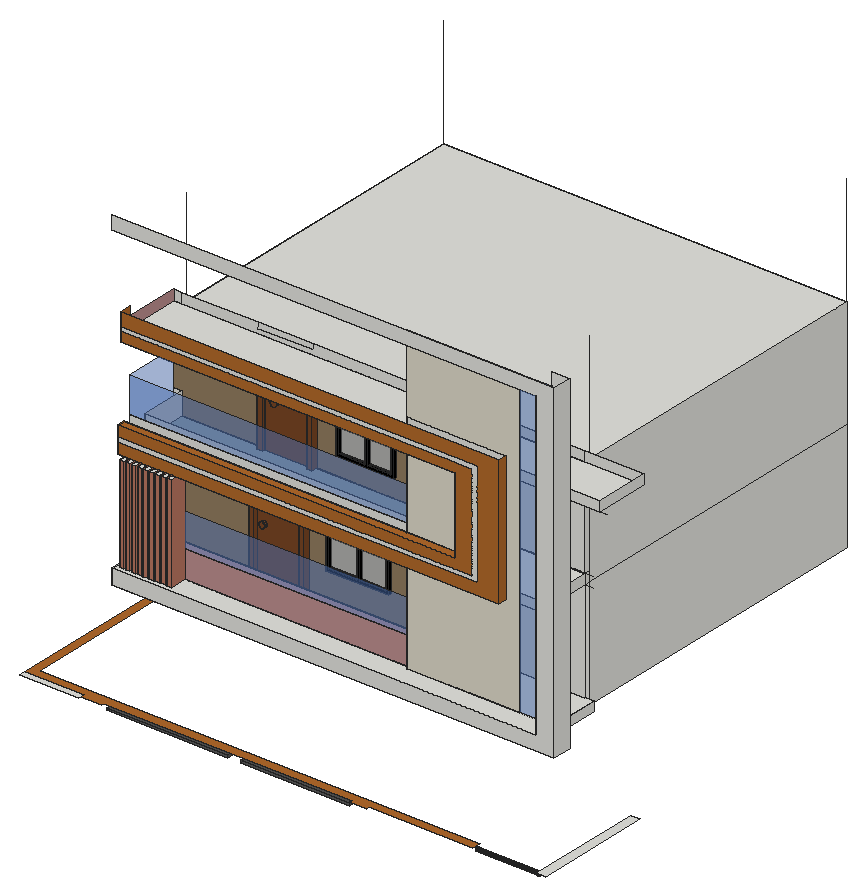
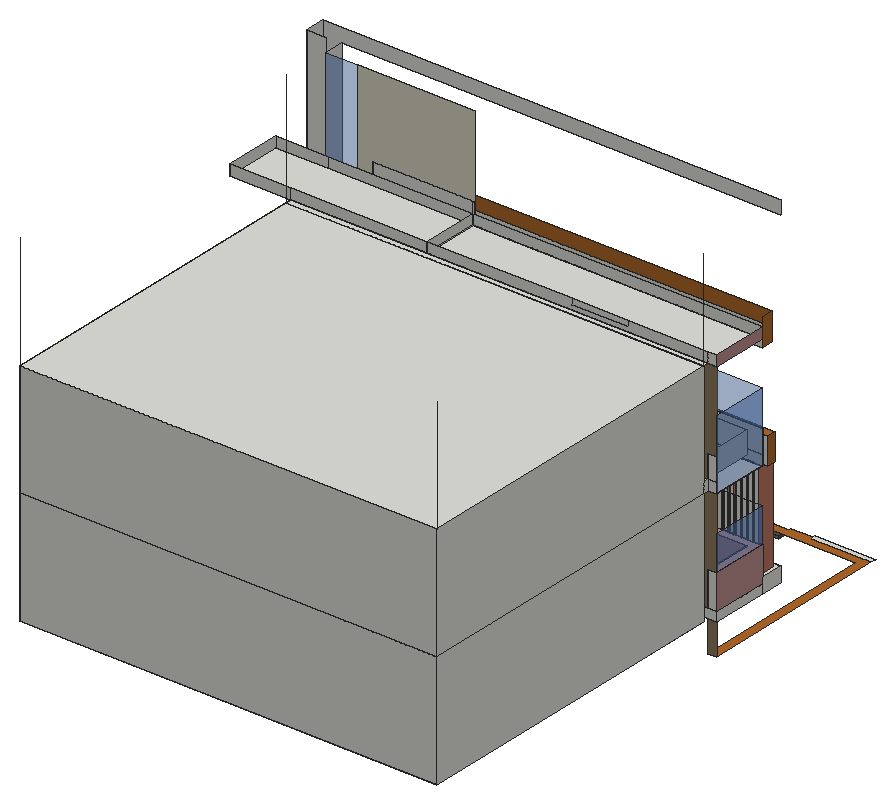
# SketchUp Ruby script. Lengths in inches.
U = 1.inch
M = Sketchup.active_model
def pt(a) = Geom::Point3d.new(a.map { |v| v * U })
def face(e, loops, mat)
  f = e.add_face(loops[0].map { |a| pt(a) })
  loops[1..].each { |l| e.add_face(l.map { |a| pt(a) }).erase! }
  f.material = f.back_material = mat if mat
  f
end
# faces: each face lists its corners as indices into pts; further lists are holes
def faces(e, pts, list, mat = nil) = list.each { |f| face(e, (f[0].is_a?(Array) ? f : [f]).map { |l| l.map { |i| pts[i] } }, mat) }
# xy, xz, yz: faces in a plane at the given z, y or x. An outline is a flat list of corners, or four numbers for a rectangle; further outlines are holes
def ring(l) = l.size == 4 ? [[l[0], l[1]], [l[2], l[1]], [l[2], l[3]], [l[0], l[3]]] : l.each_slice(2).to_a
def flat(e, list, mat, &to3) = list.each { |f| face(e, (f[0].is_a?(Array) ? f : [f]).map { |l| ring(l).map { |u, v| to3.(u, v) } }, mat) }
def xy(e, z, list, mat = nil) = flat(e, list, mat) { |x, y| [x, y, z] }
def xz(e, y, list, mat = nil) = flat(e, list, mat) { |x, z| [x, y, z] }
def yz(e, x, list, mat = nil) = flat(e, list, mat) { |y, z| [x, y, z] }
def lines(e, pts, list) = list.each { |a, b| e.add_line(pt(pts[a]), pt(pts[b])) }
# prism: a flat outline (further loops are holes) pulled along v
def prism(e, loops, v, mat = nil)
  f = face(e, loops, mat); d = Geom::Vector3d.new(v.map { |x| x * U })
  f.pushpull(f.normal.samedirection?(d) ? d.length : -d.length)
end
def box(e, o, s, mat = nil) = prism(e, [[o, [o[0] + s[0], o[1], o[2]], [o[0] + s[0], o[1] + s[1], o[2]], [o[0], o[1] + s[1], o[2]]]], [0, 0, s[2]], mat)
def at(x, y, z, deg = 0) = Geom::Transformation.translation(pt([x, y, z])) * Geom::Transformation.rotation(ORIGIN, Z_AXIS, deg.degrees)
def axes(o, x, y, z) = Geom::Transformation.new([*x, 0, *y, 0, *z, 0, *pt(o).to_a, 1])
def part(name) = M.definitions.add(name)
# library, detail: a bought-in or finely detailed component or shape, given as its bounding box
def library(name, o, s) = part(name).tap { |d| box(d.entities, o, s) }
def detail(e, o, s) = box(e.add_group.entities, o, s)
def put(e, d, t, mat = nil) = e.add_instance(d, t).tap { |i| i.material = mat if mat }
def group(e, t, mat = nil) = e.add_group.tap { |g| g.transformation = t; g.material = mat if mat }.entities
root = M.entities
M.materials.add("[0014_DarkSalmon]").color = [186, 119, 97]
M.materials.add("[0035_Tan]").color = [145, 124, 96]
M.materials.add("[0119_RosyBrown]").color = [188, 143, 143]
M.materials.add("[0135_DarkGray]").color = [81, 81, 81]
M.materials.add("[0136_Charcoal]").color = [35, 35, 35]
M.materials.add("[0137_Black]").color = [0, 0, 0]
M.materials.add("[Formica Graystone]").color = [221, 217, 201]
M.materials.add("[Marble Carrara Gold Floor Tile]").color = [225, 223, 217]
M.materials.add("[Metal Panel]").color = [143, 157, 158]
M.materials.add("[Translucent Glass Blue]").color = [90, 134, 214]
M.materials["[Translucent Glass Blue]"].alpha = 0.5
M.materials.add("[Translucent Glass Gray]").color = [128, 128, 128]
M.materials["[Translucent Glass Gray]"].alpha = 0.5
M.materials.add("[Wood Bamboo]").color = [177, 105, 43]
M.materials.add("[Wood Veneer 01]").color = [120, 70, 37]
xy(root,81.28,[[238.29,58.23,356.85,67.23]],"[0135_DarkGray]")
xy(root,81.5,[[93.07,58.23,224.96,67.23]],"[0135_DarkGray]")
xy(root,84,[[93.07,58.23,224.96,67.23],[238.29,58.23,356.85,67.23]],"[0135_DarkGray]")
xy(root,87,[[3.53,52.23,67.4,58.23],[560.78,58.23,569.78,186.0625]])
xy(root,87,[[67.4,55.23,90.07,55.23,90.07,58.23,359.85,58.23,359.85,55.23,377.85,55.23,377.85,58.23,491.3125,58.23,491.3125,67.23,12.53,67.23,12.53,261.0625,3.53,261.0625,3.53,58.23,67.4,58.23]],"[Wood Bamboo]")
xy(root,87,[[77.58,255.0625,125.58,258.0625]],"[Wood Veneer 01]")
xy(root,93,[[71.58,255.0625,131.58,261.0625]],"[Wood Veneer 01]")
xy(root,120,[[3.53,177.0625,3.53,261.0625,307.22,261.0625,307.22,198.0625,483.9,198.0625,483.9,177.0625],[307.22,198.0625,460.28,201.0625],[12.53,267.0625,450.59,616.1875]])
xy(root,129.84,[[307.22,198.0625,460.28,201.0625],[3.53,201.0625,3.53,261.0625,12.53,261.0625,12.53,210.0625,307.22,210.0625,307.22,201.0625],[307.22,201.0625,459.59,261.0625],[89.76,255.0625,95.76,261.0625],[143.76,255.0625,149.76,261.0625],
  [95.76,258.0625,143.76,261.0625]])
xy(root,129.84,[[12.53,210.0625,307.22,210.0625,307.22,261.0625,149.76,261.0625,149.76,255.0625,143.76,255.0625,143.76,258.0625,95.76,258.0625,95.76,255.0625,89.76,255.0625,89.76,261.0625,12.53,261.0625]],"[Marble Carrara Gold Floor Tile]")
xy(root,135.96,[[3.53,177.0625,464.34,177.0625,464.34,198.0625,307.22,198.0625,307.22,201.0625,63.77,201.0625,63.77,182.6875,58.71,182.6875,58.71,201.0625,57.33,201.0625,57.33,182.6875,52.27,182.6875,52.27,201.0625,50.89,201.0625,50.89,182.6875,45.83,182.6875,45.83,201.0625,44.46,201.0625,44.46,182.6875,39.39,182.6875,39.39,201.0625,38.02,201.0625,38.02,182.6875,32.96,182.6875,32.96,201.0625,31.58,201.0625,31.58,182.6875,26.52,182.6875,26.52,201.0625,25.14,201.0625,25.14,182.6875,20.08,182.6875,20.08,201.0625,18.71,201.0625,18.71,182.6875,13.64,182.6875,13.64,201.0625,12.27,201.0625,12.27,182.6875,7.21,182.6875,7.21,201.0625,3.53,201.0625],[7.21,182.6875,12.27,201.0625],[13.64,182.6875,18.71,201.0625],[20.08,182.6875,25.14,201.0625],[26.52,182.6875,31.58,201.0625],
  [32.96,182.6875,38.02,201.0625],[39.39,182.6875,44.46,201.0625],[45.83,182.6875,50.89,201.0625],[52.27,182.6875,57.33,201.0625],[58.71,182.6875,63.77,201.0625]])
xy(root,157.26,[[171.25,258.0625,239.25,261.0625]])
xy(root,160.26,[[174.25,258.0625,205.25,261.0625],[208.25,258.0625,236.25,261.0625]],"[0137_Black]")
xy(root,165.84,[[3.53,201.0625,307.22,201.0625,307.22,210.0625,12.53,210.0625,12.53,261.0625,3.53,261.0625]],"[0119_RosyBrown]")
xy(root,213.84,[[95.76,255.0625,143.76,258.0625]],"[Wood Veneer 01]")
xy(root,215.2,[[174.25,258.0625,205.25,261.0625],[208.25,258.0625,236.25,261.0625]],"[0137_Black]")
xy(root,218.2,[[171.25,258.0625,239.25,261.0625]],"[0137_Black]")
xy(root,219.84,[[89.76,255.0625,149.76,261.0625]],"[Wood Veneer 01]")
xy(root,240,[[3.53,201.0625,307.22,261.0625],[307.22,201.0625,450.59,260.625],[307.22,260.625,450.59,260.8125],[307.22,260.8125,450.59,261.0625],[12.53,261.0625,450.59,267.0625],
  [12.53,267.0625,450.59,616.1875]])
xy(root,240.5,[[7.21,182.6875,12.27,189.0625],[13.64,182.6875,18.71,189.0625],[20.08,182.6875,25.14,189.0625],[26.52,182.6875,31.58,189.0625],[32.96,182.6875,38.02,189.0625],
  [39.39,182.6875,44.46,189.0625],[45.83,182.6875,50.89,189.0625],[52.27,182.6875,57.33,189.0625],[58.71,182.6875,63.77,189.0625],[0,189.0625,7.21,198.0625],
  [7.21,189.0625,12.27,198.0625],[12.27,189.0625,13.64,198.0625],[13.64,189.0625,18.71,198.0625],[18.71,189.0625,20.08,198.0625],[20.08,189.0625,25.14,198.0625],
  [25.14,189.0625,26.52,198.0625],[26.52,189.0625,31.58,198.0625],[31.58,189.0625,32.96,198.0625],[32.96,189.0625,38.02,198.0625],[38.02,189.0625,39.39,198.0625],
  [39.39,189.0625,44.46,198.0625],[44.46,189.0625,45.83,198.0625],[45.83,189.0625,50.89,198.0625],[50.89,189.0625,52.27,198.0625],[52.27,189.0625,57.33,198.0625],
  [57.33,189.0625,58.71,198.0625],[58.71,189.0625,63.77,198.0625],[7.21,198.0625,12.27,201.0625],[13.64,198.0625,18.71,201.0625],[20.08,198.0625,25.14,201.0625],
  [26.52,198.0625,31.58,201.0625],[32.96,198.0625,38.02,201.0625],[39.39,198.0625,44.46,201.0625],[45.83,198.0625,50.89,201.0625],[52.27,198.0625,57.33,201.0625],
  [58.71,198.0625,63.77,201.0625]])
xy(root,240.5,[[63.77,189.0625,414.72,198.0625]],"[Wood Bamboo]")
xy(root,251.2,[[307.22,201.0625,450.59,260.625],[98.75,255.0625,104.75,261.0625],[152.75,255.0625,158.75,261.0625],[104.75,258.0625,152.75,261.0625],[307.22,260.625,450.59,260.8125],
  [307.22,260.8125,450.59,261.0625],[12.53,261.0625,450.59,267.0625]])
xy(root,251.2,[[12.53,210.0625,298.22,210.0625,298.22,261.0625,158.75,261.0625,158.75,255.0625,152.75,255.0625,152.75,258.0625,104.75,258.0625,104.75,255.0625,98.75,255.0625,98.75,261.0625,12.53,261.0625]],"[Metal Panel]")
xy(root,268.7,[[0,189.0625,366.75,198.0625]],"[Wood Bamboo]")
xy(root,272.3,[[181.91,258.0625,244.91,261.0625]])
xy(root,275.3,[[184.91,258.0625,213.41,261.0625],[216.41,258.0625,241.91,261.0625]],"[0137_Black]")
xy(root,330.42,[[184.91,258.0625,213.41,261.0625],[216.41,258.0625,241.91,261.0625]],"[0137_Black]")
xy(root,333.42,[[181.91,258.0625,244.91,261.0625]],"[0137_Black]")
xy(root,335.2,[[104.75,258.0625,152.75,261.0625]])
xy(root,335.2,[[104.75,255.0625,152.75,258.0625]],"[Wood Veneer 01]")
xy(root,341.2,[[98.75,255.0625,158.75,261.0625]],"[Wood Veneer 01]")
xy(root,351.4375,[[3.53,189.0625,3.53,201.0625,307.22,201.0625,307.22,198.0625,366.75,198.0625,366.75,189.0625]],"[Wood Bamboo]")
xy(root,360,[[3.53,201.0625,307.22,261.0625],[307.22,201.0625,514.15,261.0625],[12.53,261.0625,450.59,267.0625],[12.53,267.0625,450.59,616.1875]])
xz(root,177.0625,[[3.53,120,483.9,120,483.9,480,3.53,480,3.53,465.86,464.34,465.86,464.34,135.96,3.53,135.96]])
xz(root,182.6875,[[7.21,135.96,12.27,240.5],[13.64,135.96,18.71,240.5],[20.08,135.96,25.14,240.5],[26.52,135.96,31.58,240.5],[32.96,135.96,38.02,240.5],
  [39.39,135.96,44.46,240.5],[45.83,135.96,50.89,240.5],[52.27,135.96,57.33,240.5],[58.71,135.96,63.77,240.5]],"[0014_DarkSalmon]")
xz(root,189.0625,[[0,253.01,390.03,253.01,390.03,366.01,3.53,366.01,3.53,361.76,385.34,361.76,385.34,257.78,0,257.78]])
xz(root,189.0625,[[0,240.5,414.72,240.5,414.72,380.59,3.53,380.59,3.53,366.01,390.03,366.01,390.03,253.01,0,253.01],[0,257.78,385.34,257.78,385.34,361.76,3.53,361.76,3.53,351.4375,366.75,351.4375,366.75,268.7,0,268.7]],"[Wood Bamboo]")
xz(root,198.0625,[[307.22,120,400.4,129.84],[400.4,120,460.28,129.84],[460.28,120,483.9,129.84],[307.22,129.84,400.4,135.96],[400.4,129.84,460.28,135.96],
  [460.28,129.84,464.34,135.96],[464.34,129.84,483.9,182.02],[464.34,182.02,483.9,480],[0,240.5,307.22,268.7],[307.22,240.5,366.75,268.7],
  [366.75,240.5,414.72,240.5,414.72,380.59,307.22,380.59,307.22,351.4375,366.75,351.4375]])
xz(root,198.0625,[[307.22,135.96,430.34,135.96,430.34,465.86,307.22,465.86,307.22,380.59,414.72,380.59,414.72,240.5,307.22,240.5],[307.22,268.7,366.75,351.4375]],"[Formica Graystone]")
xz(root,198.0625,[[430.34,135.96,464.34,465.86]],"[Translucent Glass Blue]")
xz(root,201.0625,[[307.22,120,459.59,129.84],[3.53,129.84,307.22,135.96],[7.21,135.96,12.27,165.84],[12.27,135.96,13.64,165.84],[13.64,135.96,18.71,165.84],
  [18.71,135.96,20.08,165.84],[20.08,135.96,25.14,165.84],[25.14,135.96,26.52,165.84],[26.52,135.96,31.58,165.84],[31.58,135.96,32.96,165.84],
  [32.96,135.96,38.02,165.84],[38.02,135.96,39.39,165.84],[39.39,135.96,44.46,165.84],[44.46,135.96,45.83,165.84],[45.83,135.96,50.89,165.84],
  [50.89,135.96,52.27,165.84],[52.27,135.96,57.33,165.84],[57.33,135.96,58.71,165.84],[58.71,135.96,63.77,165.84],[7.21,165.84,12.27,202.92],
  [12.27,165.84,13.64,202.92],[13.64,165.84,18.71,202.92],[18.71,165.84,20.08,202.92],[20.08,165.84,25.14,202.92],[25.14,165.84,26.52,202.92],
  [26.52,165.84,31.58,202.92],[31.58,165.84,32.96,202.92],[32.96,165.84,38.02,202.92],[38.02,165.84,39.39,202.92],[39.39,165.84,44.46,202.92],
  [44.46,165.84,45.83,202.92],[45.83,165.84,50.89,202.92],[50.89,165.84,52.27,202.92],[52.27,165.84,57.33,202.92],[57.33,165.84,58.71,202.92],
  [58.71,165.84,63.77,202.92],[7.21,202.92,12.27,240],[13.64,202.92,18.71,240],[20.08,202.92,25.14,240],[26.52,202.92,31.58,240],
  [32.96,202.92,38.02,240],[39.39,202.92,44.46,240],[45.83,202.92,50.89,240],[52.27,202.92,57.33,240],[58.71,202.92,63.77,240],
  [3.53,240,7.21,240,7.21,240.5,12.27,240.5,12.27,240,13.64,240,13.64,240.5,18.71,240.5,18.71,240,20.08,240,20.08,240.5,25.14,240.5,25.14,240,26.52,240,26.52,240.5,31.58,240.5,31.58,240,32.96,240,32.96,240.5,38.02,240.5,38.02,240,39.39,240,39.39,240.5,44.46,240.5,44.46,240,45.83,240,45.83,240.5,50.89,240.5,50.89,240,52.27,240,52.27,240.5,57.33,240.5,57.33,240,58.71,240,58.71,240.5,63.77,240.5,63.77,240,307.22,240,307.22,251.2,3.53,251.2],[7.21,240,12.27,240.5],[13.64,240,18.71,240.5],[20.08,240,25.14,240.5],[26.52,240,31.58,240.5],
  [32.96,240,38.02,240.5],[39.39,240,44.46,240.5],[45.83,240,50.89,240.5],[52.27,240,57.33,240.5],[58.71,240,63.77,240.5],
  [307.22,240,450.59,251.2],[3.53,251.2,307.22,275.2],[3.53,351.4375,307.22,360],[3.53,360,307.22,370.9],[307.22,360,459.59,370.9],
  [459.59,360,514.15,370.9]])
xz(root,201.0625,[[3.53,135.96,7.21,165.84],[63.77,135.96,307.22,165.84]],"[0119_RosyBrown]")
xz(root,201.0625,[[3.53,165.84,7.21,202.92],[63.77,165.84,307.22,202.92],[3.53,275.2,307.22,313.68]],"[Translucent Glass Blue]")
xz(root,210.0625,[[12.53,251.2,298.22,275.2]])
xz(root,210.0625,[[12.53,129.84,307.22,165.84]],"[0119_RosyBrown]")
xz(root,255.0625,[[89.76,129.84,95.76,129.84,95.76,213.84,143.76,213.84,143.76,129.84,149.76,129.84,149.76,219.84,89.76,219.84],[103.85,175.78,104.66,175.84,105.43,176.12,106.1,176.58,106.63,177.21,106.98,177.95,107.12,178.75,107.05,179.5625,106.78,180.33,106.3125,181,105.69,181.53,104.95,181.875,104.15,182.02,103.34,181.95,102.57,181.67,101.9,181.21,101.37,180.59,101.02,179.85,100.88,179.05,100.95,178.23,101.22,177.47,101.6875,176.8,102.31,176.27,103.05,175.92],[98.75,251.2,104.75,251.2,104.75,335.2,152.75,335.2,152.75,251.2,158.75,251.2,158.75,341.2,98.75,341.2],[116.3,298.54,117.42,298.69,118.46,299.12,119.35,299.81,120.03,300.7,120.47,301.74,120.61,302.86,120.47,303.97,120.03,305.01,119.35,305.91,118.46,306.59,117.42,307.02,116.3,307.17,115.18,307.02,114.14,306.59,113.25,305.91,112.57,305.01,112.13,303.97,111.99,302.86,112.13,301.74,112.57,300.7,113.25,299.81,114.14,299.12,115.18,298.69]],"[Wood Veneer 01]")
xz(root,258.0625,[[103.85,175.78,103.05,175.92,102.31,176.27,101.6875,176.8,101.22,177.47,100.95,178.23,100.88,179.05,101.02,179.85,101.37,180.59,101.9,181.21,102.57,181.67,103.34,181.95,104.15,182.02,104.95,181.875,105.69,181.53,106.3125,181,106.78,180.33,107.05,179.5625,107.12,178.75,106.98,177.95,106.63,177.21,106.1,176.58,105.43,176.12,104.66,175.84],[116.3,298.54,115.18,298.69,114.14,299.12,113.25,299.81,112.57,300.7,112.13,301.74,111.99,302.86,112.13,303.97,112.57,305.01,113.25,305.91,114.14,306.59,115.18,307.02,116.3,307.17,117.42,307.02,118.46,306.59,119.35,305.91,120.03,305.01,120.47,303.97,120.61,302.86,120.47,301.74,120.03,300.7,119.35,299.81,118.46,299.12,117.42,298.69]])
xz(root,258.0625,[[[171.25,157.26,239.25,218.2],[174.25,160.26,205.25,215.2],[208.25,160.26,236.25,215.2]],[[181.91,272.3,244.91,333.42],[184.91,275.3,213.41,330.42],[216.41,275.3,241.91,330.42]]],"[0137_Black]")
xz(root,258.0625,[[[95.76,129.84,143.76,213.84],[103.85,175.78,103.05,175.92,102.31,176.27,101.6875,176.8,101.22,177.47,100.95,178.23,100.88,179.05,101.02,179.85,101.37,180.59,101.9,181.21,102.57,181.67,103.34,181.95,104.15,182.02,104.95,181.875,105.69,181.53,106.3125,181,106.78,180.33,107.05,179.5625,107.12,178.75,106.98,177.95,106.63,177.21,106.1,176.58,105.43,176.12,104.66,175.84]],[[104.75,251.2,152.75,335.2],[116.3,298.54,115.18,298.69,114.14,299.12,113.25,299.81,112.57,300.7,112.13,301.74,111.99,302.86,112.13,303.97,112.57,305.01,113.25,305.91,114.14,306.59,115.18,307.02,116.3,307.17,117.42,307.02,118.46,306.59,119.35,305.91,120.03,305.01,120.47,303.97,120.61,302.86,120.47,301.74,120.03,300.7,119.35,299.81,118.46,299.12,117.42,298.69]]],"[Wood Veneer 01]")
xz(root,260.625,[[307.22,240,450.59,251.2]])
xz(root,260.8125,[[307.22,240,450.59,251.2]])
xz(root,261.0625,[[3.53,120,307.22,120,307.22,129.84,149.76,129.84,149.76,123.84,89.76,123.84,89.76,129.84,3.53,129.84],[89.76,123.84,149.76,129.84],[3.53,129.84,12.53,165.84],[307.22,129.84,450.59,240],[3.53,240,12.53,251.2],
  [12.53,240,12.53,251.2,98.75,251.2,98.75,245.2,158.75,245.2,158.75,251.2,307.22,251.2,307.22,240],[307.22,240,450.59,251.2],[98.75,245.2,158.75,251.2],[3.53,251.2,12.53,275.2],[98.75,251.2,98.75,341.2,158.75,341.2,158.75,251.2,152.75,251.2,152.75,335.2,104.75,335.2,104.75,251.2],
  [298.22,251.2,307.22,275.2],[307.22,251.2,450.59,360],[[181.91,272.3,244.91,333.42],[184.91,275.3,213.41,330.42],[216.41,275.3,241.91,330.42]],[3.53,360,12.53,370.9],[12.53,360,12.53,370.9,95.3,370.9,95.3,364.9,155.3,364.9,155.3,370.9,307.22,370.9,307.22,360],
  [307.22,360,450.59,370.9],[450.59,360,514.15,370.9],[95.3,364.9,155.3,370.9]])
xz(root,261.0625,[[3.53,87,12.53,120],[[12.53,129.84,89.76,129.84,89.76,219.84,149.76,219.84,149.76,129.84,307.22,129.84,307.22,240,3.53,240,3.53,165.84,12.53,165.84],[171.25,157.26,239.25,218.2]],[[12.53,251.2,98.75,251.2,98.75,341.2,158.75,341.2,158.75,251.2,298.22,251.2,298.22,275.2,307.22,275.2,307.22,360,3.53,360,3.53,275.2,12.53,275.2],[181.91,272.3,244.91,333.42]]],"[0035_Tan]")
xz(root,261.0625,[[174.25,160.26,205.25,215.2],[208.25,160.26,236.25,215.2],[184.91,275.3,213.41,330.42],[216.41,275.3,241.91,330.42]],"[Translucent Glass Gray]")
xz(root,267.0625,[[12.53,120,450.59,240],[12.53,240,450.59,251.2],[12.53,251.2,450.59,360]])
xz(root,616.1875,[[12.53,120,450.59,240],[12.53,240,450.59,360]])
yz(root,0,[[189.0625,240.5,198.0625,268.7]],"[Wood Bamboo]")
yz(root,3.53,[[177.0625,120,201.0625,135.96],[201.0625,120,261.0625,129.84]])
yz(root,3.53,[[201.0625,129.84,261.0625,165.84],[201.0625,360,261.0625,370.9]],"[0119_RosyBrown]")
yz(root,3.53,[[201.0625,165.84,261.0625,202.92],[201.0625,240,261.0625,313.68]],"[Translucent Glass Blue]")
yz(root,3.53,[[189.0625,351.4375,201.0625,380.59]],"[Wood Bamboo]")
yz(root,7.21,[[182.6875,135.96,201.0625,240.5]],"[0014_DarkSalmon]")
yz(root,12.27,[[182.6875,135.96,201.0625,240.5]],"[0014_DarkSalmon]")
yz(root,12.53,[[267.0625,120,616.1875,240],[261.0625,240,267.0625,251.2],[267.0625,240,616.1875,360],[210.0625,251.2,261.0625,275.2]])
yz(root,12.53,[[210.0625,129.84,261.0625,165.84]],"[0119_RosyBrown]")
yz(root,13.64,[[182.6875,135.96,201.0625,240.5]],"[0014_DarkSalmon]")
yz(root,18.71,[[182.6875,135.96,201.0625,240.5]],"[0014_DarkSalmon]")
yz(root,20.08,[[182.6875,135.96,201.0625,240.5]],"[0014_DarkSalmon]")
yz(root,25.14,[[182.6875,135.96,201.0625,240.5]],"[0014_DarkSalmon]")
yz(root,26.52,[[182.6875,135.96,201.0625,240.5]],"[0014_DarkSalmon]")
yz(root,31.58,[[182.6875,135.96,201.0625,240.5]],"[0014_DarkSalmon]")
yz(root,32.96,[[182.6875,135.96,201.0625,240.5]],"[0014_DarkSalmon]")
yz(root,38.02,[[182.6875,135.96,201.0625,240.5]],"[0014_DarkSalmon]")
yz(root,39.39,[[182.6875,135.96,201.0625,240.5]],"[0014_DarkSalmon]")
yz(root,44.46,[[182.6875,135.96,201.0625,240.5]],"[0014_DarkSalmon]")
yz(root,45.83,[[182.6875,135.96,201.0625,240.5]],"[0014_DarkSalmon]")
yz(root,50.89,[[182.6875,135.96,201.0625,240.5]],"[0014_DarkSalmon]")
yz(root,52.27,[[182.6875,135.96,201.0625,240.5]],"[0014_DarkSalmon]")
yz(root,57.33,[[182.6875,135.96,201.0625,240.5]],"[0014_DarkSalmon]")
yz(root,58.71,[[182.6875,135.96,201.0625,240.5]],"[0014_DarkSalmon]")
yz(root,63.77,[[182.6875,135.96,201.0625,240.5]],"[0014_DarkSalmon]")
yz(root,89.76,[[255.0625,129.84,261.0625,219.84]],"[Wood Veneer 01]")
yz(root,93.07,[[58.23,81.5,67.23,84]],"[0135_DarkGray]")
yz(root,95.76,[[255.0625,129.84,258.0625,213.84]],"[Wood Veneer 01]")
yz(root,98.75,[[255.0625,251.2,261.0625,341.2]],"[Wood Veneer 01]")
yz(root,104.75,[[258.0625,251.2,261.0625,335.2]])
yz(root,104.75,[[255.0625,251.2,258.0625,335.2]],"[Wood Veneer 01]")
yz(root,143.76,[[255.0625,129.84,258.0625,213.84]],"[Wood Veneer 01]")
yz(root,149.76,[[255.0625,129.84,261.0625,219.84]],"[Wood Veneer 01]")
yz(root,152.75,[[258.0625,251.2,261.0625,335.2]])
yz(root,152.75,[[255.0625,251.2,258.0625,335.2]],"[Wood Veneer 01]")
yz(root,158.75,[[255.0625,251.2,261.0625,341.2]],"[Wood Veneer 01]")
yz(root,171.25,[[258.0625,157.26,261.0625,218.2]])
yz(root,174.25,[[258.0625,160.26,261.0625,215.2]],"[0137_Black]")
yz(root,181.91,[[258.0625,272.3,261.0625,333.42]],"[0137_Black]")
yz(root,184.91,[[258.0625,275.3,261.0625,330.42]],"[0137_Black]")
yz(root,205.25,[[258.0625,160.26,261.0625,215.2]])
yz(root,208.25,[[258.0625,160.26,261.0625,215.2]],"[0137_Black]")
yz(root,213.41,[[258.0625,275.3,261.0625,330.42]],"[0137_Black]")
yz(root,216.41,[[258.0625,275.3,261.0625,330.42]],"[0137_Black]")
yz(root,224.96,[[58.23,81.5,67.23,84]],"[0135_DarkGray]")
yz(root,236.25,[[258.0625,160.26,261.0625,215.2]],"[0137_Black]")
yz(root,238.29,[[58.23,81.28,67.23,84]],"[0135_DarkGray]")
yz(root,239.25,[[258.0625,157.26,261.0625,218.2]],"[0137_Black]")
yz(root,241.91,[[258.0625,275.3,261.0625,330.42]],"[0137_Black]")
yz(root,244.91,[[258.0625,272.3,261.0625,333.42]],"[0137_Black]")
yz(root,298.22,[[210.0625,251.2,261.0625,275.2]])
yz(root,307.22,[[198.0625,120,201.0625,129.84],[201.0625,120,261.0625,129.84],[198.0625,129.84,201.0625,135.96],[201.0625,129.84,210.0625,165.84],[210.0625,129.84,210.0625,165.84,201.0625,165.84,201.0625,240,261.0625,240,261.0625,129.84],
  [198.0625,135.96,201.0625,351.4375],[201.0625,240,260.625,251.2],[260.625,240,260.8125,251.2],[260.8125,240,261.0625,251.2],[201.0625,251.2,260.625,275.2],
  [260.625,251.2,260.8125,275.2],[260.8125,251.2,261.0625,275.2],[201.0625,275.2,261.0625,360],[198.0625,351.4375,200.5,380.59],[200.5,351.4375,201.0625,380.59],
  [201.0625,360,261.0625,370.9]])
yz(root,356.85,[[58.23,81.28,67.23,84]],"[0135_DarkGray]")
yz(root,366.75,[[189.0625,268.7,198.0625,351.4375]],"[Wood Bamboo]")
yz(root,414.72,[[189.0625,240.5,198.0625,380.59]],"[Wood Bamboo]")
yz(root,450.59,[[267.0625,120,616.1875,240],[201.0625,240,260.625,251.2],[260.625,240,260.8125,251.2],[260.8125,240,261.0625,251.2],[261.0625,240,267.0625,251.2],
  [267.0625,240,616.1875,360],[261.0625,251.2,267.0625,360]])
yz(root,460.28,[[198.0625,120,261.0625,129.84]])
yz(root,464.34,[[177.0625,135.96,198.0625,465.86]])
yz(root,483.9,[[177.0625,120,198.0625,480]])
yz(root,514.15,[[201.0625,360,261.0625,370.9]])
p = [[491.3125,62.4,82.66],[491.3125,62.8,82.6],[560.78,62.8,82.6],[560.78,62.4,82.66],[491.3125,63.2,82.66],[560.78,63.2,82.66],
  [491.3125,62.02,82.8125],[560.78,62.02,82.8125],[491.3125,63.58,82.8125],[560.78,63.58,82.8125],[491.3125,61.7,83.0625],[560.78,61.7,83.0625],
  [491.3125,63.91,83.0625],[560.78,63.91,83.0625],[491.3125,61.45,83.39],[560.78,61.45,83.39],[491.3125,64.15,83.39],[560.78,64.15,83.39],
  [491.3125,61.29,83.76],[560.78,61.29,83.76],[491.3125,64.31,83.76],[560.78,64.31,83.76],[491.3125,61.24,84.17],[560.78,61.24,84.17],
  [491.3125,64.36,84.17],[560.78,64.36,84.17],[491.3125,61.29,84.57],[560.78,61.29,84.57],[491.3125,64.31,84.57],[560.78,64.31,84.57],
  [491.3125,61.45,84.95],[560.78,61.45,84.95],[491.3125,64.15,84.95],[560.78,64.15,84.95],[491.3125,61.7,85.27],[560.78,61.7,85.27],
  [491.3125,63.91,85.27],[560.78,63.91,85.27],[491.3125,62.02,85.52],[560.78,62.02,85.52],[491.3125,63.58,85.52],[560.78,63.58,85.52],
  [491.3125,62.4,85.68],[560.78,62.4,85.68],[491.3125,63.2,85.68],[560.78,63.2,85.68],[491.3125,62.8,85.73],[560.78,62.8,85.73],
  [103.05,258.0625,175.92],[103.85,258.0625,175.78],[103.85,255.0625,175.78],[103.05,255.0625,175.92],[104.66,258.0625,175.84],[104.66,255.0625,175.84],
  [105.43,258.0625,176.12],[105.43,255.0625,176.12],[102.31,258.0625,176.27],[102.31,255.0625,176.27],[106.1,258.0625,176.58],[106.1,255.0625,176.58],
  [101.6875,258.0625,176.8],[101.6875,255.0625,176.8],[106.63,258.0625,177.21],[106.63,255.0625,177.21],[101.22,258.0625,177.47],[101.22,255.0625,177.47],
  [106.98,258.0625,177.95],[106.98,255.0625,177.95],[100.95,258.0625,178.23],[100.95,255.0625,178.23],[107.12,258.0625,178.75],[107.12,255.0625,178.75],
  [100.88,258.0625,179.05],[100.88,255.0625,179.05],[107.05,258.0625,179.5625],[107.05,255.0625,179.5625],[101.02,258.0625,179.85],[101.02,255.0625,179.85],
  [106.78,258.0625,180.33],[106.78,255.0625,180.33],[101.37,258.0625,180.59],[101.37,255.0625,180.59],[106.3125,258.0625,181],[106.3125,255.0625,181],
  [101.9,258.0625,181.21],[101.9,255.0625,181.21],[105.69,258.0625,181.53],[105.69,255.0625,181.53],[102.57,258.0625,181.67],[102.57,255.0625,181.67],
  [104.95,258.0625,181.875],[104.95,255.0625,181.875],[103.34,258.0625,181.95],[103.34,255.0625,181.95],[104.15,258.0625,182.02],[104.15,255.0625,182.02],
  [115.18,258.0625,298.69],[116.3,258.0625,298.54],[116.3,255.0625,298.54],[115.18,255.0625,298.69],[117.42,258.0625,298.69],[117.42,255.0625,298.69],
  [114.14,258.0625,299.12],[114.14,255.0625,299.12],[118.46,258.0625,299.12],[118.46,255.0625,299.12],[113.25,258.0625,299.81],[113.25,255.0625,299.81],
  [119.35,258.0625,299.81],[119.35,255.0625,299.81],[112.57,258.0625,300.7],[112.57,255.0625,300.7],[120.03,258.0625,300.7],[120.03,255.0625,300.7],
  [112.13,258.0625,301.74],[112.13,255.0625,301.74],[120.47,258.0625,301.74],[120.47,255.0625,301.74],[111.99,258.0625,302.86],[111.99,255.0625,302.86],
  [120.61,258.0625,302.86],[120.61,255.0625,302.86],[112.13,258.0625,303.97],[112.13,255.0625,303.97],[120.47,258.0625,303.97],[120.47,255.0625,303.97],
  [112.57,258.0625,305.01],[112.57,255.0625,305.01],[120.03,258.0625,305.01],[120.03,255.0625,305.01],[113.25,258.0625,305.91],[113.25,255.0625,305.91],
  [119.35,258.0625,305.91],[119.35,255.0625,305.91],[114.14,258.0625,306.59],[114.14,255.0625,306.59],[118.46,258.0625,306.59],[118.46,255.0625,306.59],
  [115.18,258.0625,307.02],[115.18,255.0625,307.02],[117.42,258.0625,307.02],[117.42,255.0625,307.02],[116.3,258.0625,307.17],[116.3,255.0625,307.17],
  [12.53,616.1875,360],[12.53,616.1875,480],[12.53,267.0625,360],[12.53,267.0625,465.86],[450.59,616.1875,360],[450.59,616.1875,480],
  [450.59,267.0625,360],[450.59,267.0625,480],[459.59,261.0625,251.2],[450.59,261.0625,251.2],[459.59,201.0625,251.2],[450.59,201.0625,251.2],
  [450.59,261.0625,240],[459.59,261.0625,240],[459.59,237.0625,129.84],[459.59,237.0625,120],[514.15,201.0625,360],[522.97,201.0625,360]]
faces(root,p,[[0,1,2,3],[1,4,5,2],[6,0,3,7],[4,8,9,5],[10,6,7,11],[8,12,13,9],[14,10,11,15],[12,16,17,13],
  [18,14,15,19],[16,20,21,17],[22,18,19,23],[20,24,25,21],[26,22,23,27],[24,28,29,25],[30,26,27,31],[28,32,33,29],
  [34,30,31,35],[32,36,37,33],[38,34,35,39],[36,40,41,37],[42,38,39,43],[40,44,45,41],[46,42,43,47],[44,46,47,45]],"[0136_Charcoal]")
faces(root,p,[[48,49,50,51],[49,52,53,50],[52,54,55,53],[56,48,51,57],[54,58,59,55],[60,56,57,61],[58,62,63,59],[64,60,61,65],
  [62,66,67,63],[68,64,65,69],[66,70,71,67],[72,68,69,73],[70,74,75,71],[76,72,73,77],[74,78,79,75],[80,76,77,81],
  [78,82,83,79],[84,80,81,85],[82,86,87,83],[88,84,85,89],[86,90,91,87],[92,88,89,93],[90,94,95,91],[94,92,93,95],
  [96,97,98,99],[97,100,101,98],[102,96,99,103],[100,104,105,101],[106,102,103,107],[104,108,109,105],[110,106,107,111],[108,112,113,109],
  [114,110,111,115],[112,116,117,113],[118,114,115,119],[116,120,121,117],[122,118,119,123],[120,124,125,121],[126,122,123,127],[124,128,129,125],
  [130,126,127,131],[128,132,133,129],[134,130,131,135],[132,136,137,133],[138,134,135,139],[136,140,141,137],[142,138,139,143],[140,142,143,141]],"[Wood Veneer 01]")
lines(root,p,[[144,145],[146,147],[148,149],[150,151],[152,153],[154,155],[156,157],[158,159],[160,161]])
